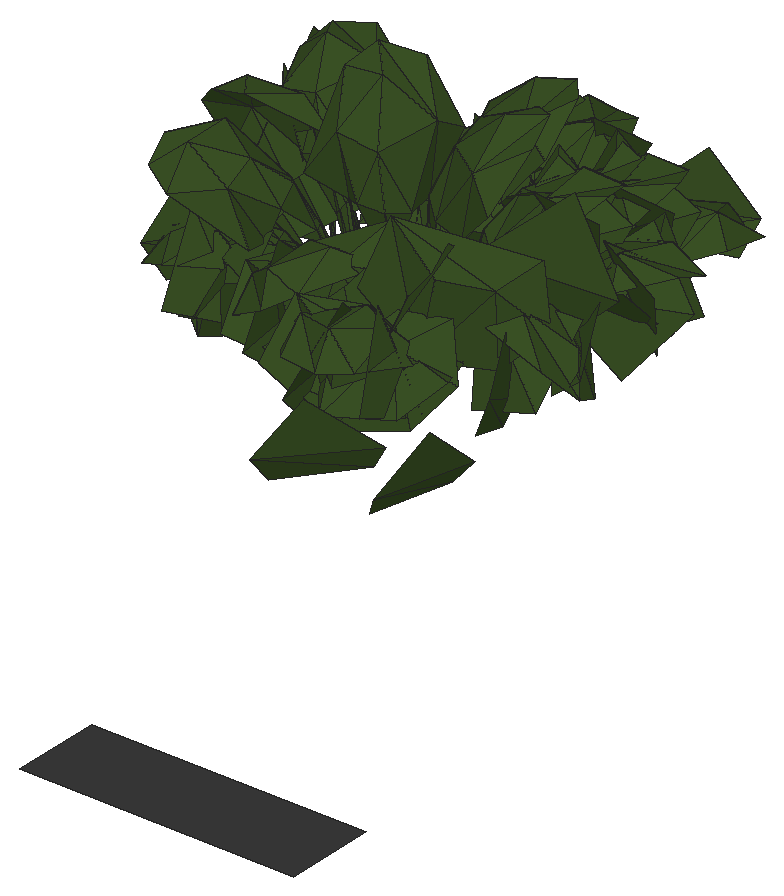
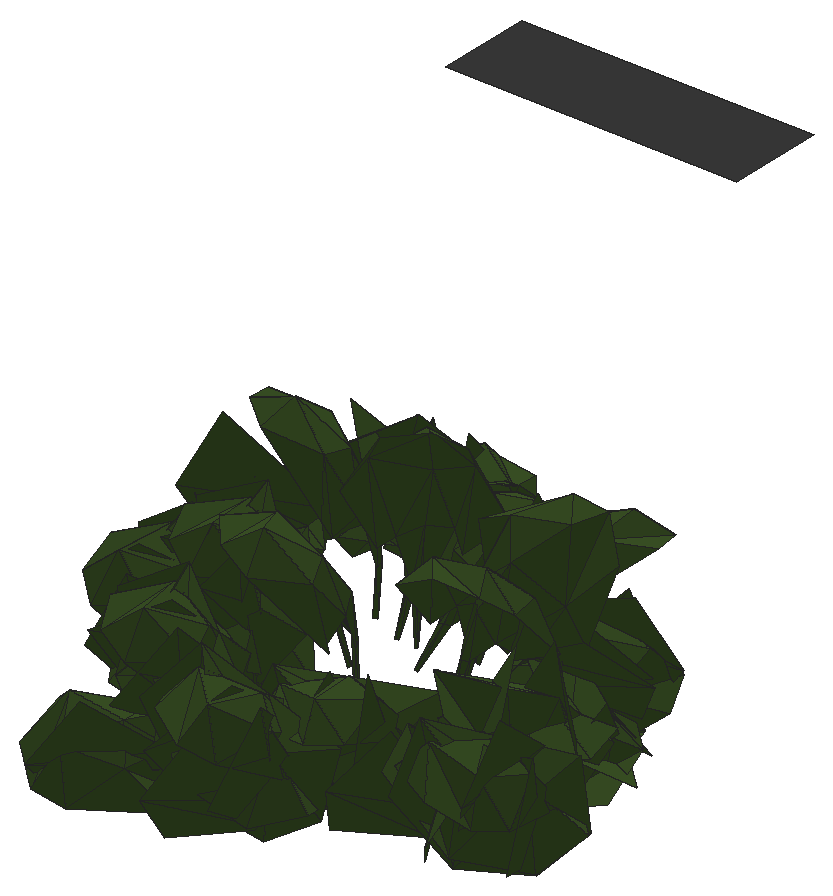
# SketchUp Ruby script. Lengths in inches.
U = 1.inch
M = Sketchup.active_model
def pt(a) = Geom::Point3d.new(a.map { |v| v * U })
def face(e, loops, mat)
  f = e.add_face(loops[0].map { |a| pt(a) })
  loops[1..].each { |l| e.add_face(l.map { |a| pt(a) }).erase! }
  f.material = f.back_material = mat if mat
  f
end
# faces: each face lists its corners as indices into pts; further lists are holes
def faces(e, pts, list, mat = nil) = list.each { |f| face(e, (f[0].is_a?(Array) ? f : [f]).map { |l| l.map { |i| pts[i] } }, mat) }
# xy, xz, yz: faces in a plane at the given z, y or x. An outline is a flat list of corners, or four numbers for a rectangle; further outlines are holes
def ring(l) = l.size == 4 ? [[l[0], l[1]], [l[2], l[1]], [l[2], l[3]], [l[0], l[3]]] : l.each_slice(2).to_a
def flat(e, list, mat, &to3) = list.each { |f| face(e, (f[0].is_a?(Array) ? f : [f]).map { |l| ring(l).map { |u, v| to3.(u, v) } }, mat) }
def xy(e, z, list, mat = nil) = flat(e, list, mat) { |x, y| [x, y, z] }
def xz(e, y, list, mat = nil) = flat(e, list, mat) { |x, z| [x, y, z] }
def yz(e, x, list, mat = nil) = flat(e, list, mat) { |y, z| [x, y, z] }
def lines(e, pts, list) = list.each { |a, b| e.add_line(pt(pts[a]), pt(pts[b])) }
# prism: a flat outline (further loops are holes) pulled along v
def prism(e, loops, v, mat = nil)
  f = face(e, loops, mat); d = Geom::Vector3d.new(v.map { |x| x * U })
  f.pushpull(f.normal.samedirection?(d) ? d.length : -d.length)
end
def box(e, o, s, mat = nil) = prism(e, [[o, [o[0] + s[0], o[1], o[2]], [o[0] + s[0], o[1] + s[1], o[2]], [o[0], o[1] + s[1], o[2]]]], [0, 0, s[2]], mat)
def at(x, y, z, deg = 0) = Geom::Transformation.translation(pt([x, y, z])) * Geom::Transformation.rotation(ORIGIN, Z_AXIS, deg.degrees)
def axes(o, x, y, z) = Geom::Transformation.new([*x, 0, *y, 0, *z, 0, *pt(o).to_a, 1])
def part(name) = M.definitions.add(name)
# library, detail: a bought-in or finely detailed component or shape, given as its bounding box
def library(name, o, s) = part(name).tap { |d| box(d.entities, o, s) }
def detail(e, o, s) = box(e.add_group.entities, o, s)
def put(e, d, t, mat = nil) = e.add_instance(d, t).tap { |i| i.material = mat if mat }
def group(e, t, mat = nil) = e.add_group.tap { |g| g.transformation = t; g.material = mat if mat }.entities
root = M.entities
M.materials.add("AM113_062_Tilia").color = [58, 81, 37]
M.materials.add("[Color M07]").color = [58, 58, 58]
xy(root,690.29,[[622.42,139.5,935.92,242.3125]],"[Color M07]")
p = [[327.63,1139.99,685.84],[309.71,1220.66,616.22],[297.98,1281.88,690],[174.23,954.27,619.67],[231,919.16,655.06],[205.29,943.34,722.98],
  [154.57,967.09,702.43],[140.39,1031,708.31],[108.83,998.61,649.08],[307.93,1122,668.52],[310.69,1104.29,621.81],[311.32,1108.2,619.89],
  [311.49,1128.11,668.52],[303.43,1122.55,663.09],[308.5,1107.52,620.19],[389.02,759.99,653.48],[390.55,785.18,622.06],[464.66,843.46,635.39],
  [420.88,1218.61,654.95],[420.67,1190.75,623.84],[419.95,1187.76,627.35],[395.14,1156.22,667.875],[395.59,1141.64,624.24],[393.67,1138.13,625.47],
  [83.33,1185.82,624.62],[56.51,1146.41,657.09],[82.44,1189.61,706.24],[130.1,1239.65,638.93],[395.65,1152.44,674.15],[397.61,1139.62,624.95],
  [402.38,1152.74,676.91],[423.08,1217.59,662.28],[423.24,1189.62,624.87],[429.7,1220.08,662.4375],[381.2,1345.93,663.1875],[365.77,1332.66,626.33],
  [280.68,1294.44,648.45],[550.8,901.41,709.43],[536.91,899.74,667.9375],[501.37,982.28,628.85],[500.73,1003.03,649.21],[185.51,1160.68,715.51],
  [167.09,1230.71,629.01],[121.44,1288.29,683.09],[187.5,1196.21,629.25],[174.67,1183.04,653.09],[228.74,1287.03,699.15],[233.375,1276.51,656.4],
  [70.38,1206.76,751.58],[90.97,1167.86,632.32],[164.75,1148.38,699.71],[70.45,1240.96,653.14],[413.95,1326.36,673.74],[381.95,1306.6875,632.77],
  [411.5625,1271.92,633.99],[447.59,1363.01,639.1875],[382.33,938.86,709.29],[393.79,860.28,633.7],[399.17,794.95,702.68],[562.03,1126.64,659.14],
  [518.35,1180.6,633.72],[509.52,1180.36,714.6875],[478.72,1212.45,656.82],[533.04,757.23,664.18],[513.99,775.86,634.76],[535.22,868.29,634.04],
  [552.33,878.07,656.07],[408.8,1270.31,671.65],[155.32,950.27,634.76],[208.75,906.27,669.96],[209.82,955.9375,720.57],[179.46,1062.71,668.15],
  [120.11,1023.59,651.5],[169,992.7,700.77],[147.91,1120.65,634.8],[83.88,1089.46,650.38],[108.71,1011.38,661.23],[136.75,1065.66,699.34],
  [176.39,1030.09,725.68],[247.48,1021.8125,698.34],[480.53,841.21,661.92],[325.08,1197.39,676.07],[332.71,1179.9,635.42],[333.03,1176.14,637.49],
  [298.78,993.79,708.55],[327.84,918.16,635.86],[309.45,849.57,695.18],[275.48,1041.15,635.88],[245.66,1034.51,674.23],[252.27,1034.3,677.43],
  [278.5,1042.57,639.24],[327.67,1195.35,682.82],[335.52,1179.4,636.17],[333.19,1199.55,684.54],[520.78,1189.57,764.04],[498.7,1175.5,636.34],
  [459.35,1104.71,693.92],[569.19,1185.41,676.24],[255.2,1029.8,673.47],[277.17,1039.02,637.22],[285.36,1300.09,637.23],[239.24,1281.06,663.58],
  [285.0625,1291.0625,718.17],[354.96,1310.96,657.4375],[448.375,1097.28,678.25],[437.37,1080.01,638.73],[434.24,1077.97,640.92],[113.56,1236.78,724.35],
  [169.17,1235.62,769.29],[162.83,1285.08,716.625],[467.15,1346.8,686.42],[482.3125,1367.17,647.91],[488.72,1366.5625,669],[485.34,1340.26,639.38],
  [407.73,1287.54,657.32],[447.81,1094.35,685.24],[438.32,1077.37,639.72],[454.17,1091.73,687.29],[285.01,1304.65,767.97],[280.18,1280.45,639.78],
  [324.8125,1210.37,692.13],[308.38,1345.99,679.18],[67.85,1205.9,640.49],[47.12,1160.9,665.06],[94.26,1183.34,708.76],[122.28,1254.76,658.12],
  [348.37,1204.82,707.76],[378.88,1283.14,641.04],[376.96,1346.91,712.72],[124.99,1008.1875,641.44],[182.85,975.625,677.9],[171.24,1019.73,734.7],
  [113.64,1107.77,694.77],[70.23,1067.42,662.12],[120.66,1044.59,715.81],[281.19,1237.625,642.22],[220.04,1199.44,646.54],[240.28,1194.91,723.81],
  [286.29,1230.3,729.59],[347.3,1210.41,747.36],[342.74,1264.82,703.2],[466.02,1082.3125,711.53],[549.87,1091.34,645.39],[603.58,1128.0625,715.14],
  [441.98,1023.9,736.48],[479.3125,965.46,645.89],[560.48,955.8125,674.03],[402.16,972.05,646.15],[399.66,950.03,693.13],[403.75,955.78,693.65],
  [403.11,975.8,648.38],[408.24,955.09,688.24],[405.03,972.46,646.53],[192.5,1165.17,686.79],[495.4,1297.59,708.6875],[514.02,1341.27,670.84],
  [271.59,1292.72,679.9],[411.16,1257.73,780.51],[404.89,1253.14,648.81],[400.51,1165.51,686.49],[460.25,1288.15,702.5],[521.99,960.06,741.96],
  [245.33,1209.74,772.58],[223.73,1179.5,649.5],[301.47,1135.125,679.47],[231.03,1252.6,681.81],[482.41,1235.93,674.75],[419.9375,1266.85,650.66],
  [408.1,1251.43,728.49],[368.9,1273.55,671.32],[174.04,1136.39,687.26],[193.76,1122.12,651.58],[196.14,1119.7,654.56],[149.86,1087.9,725.7],
  [104.32,1050.1,700.87],[162,1041.35,652.08],[238.74,1163.21,699.8125],[176.82,1137.3125,694.29],[196.22,1123.5625,652.34],[178.49,1144.17,694.7],
  [206.1,1228.36,738.91],[415.99,1146.52,701.32],[488.98,1201.49,653.22],[515.44,1248.21,737.56],[430.64,785.71,718.13],[397.04,1061.99,697.77],
  [397.28,1047.24,654.22],[394.88,1044.02,655.33],[228.125,1119.78,672.11],[150.4,1179.01,654.22],[119.5,1191.48,754.53],[425.14,1255.45,693],
  [260.47,913.6,712.85],[396.8,1058.21,704.08],[399,1044.97,655.06],[403.4,1057.64,707.27],[574.78,1132.12,682.14],[537.48,1192.99,655.09],
  [501.4375,1169.52,715.01],[492.82,1219.65,668.76],[150.6875,1034.22,776.35],[199.36,987.61,676.91],[207.05,1078.21,655.21],[571.36,1026.58,662.9],
  [508.7,1086.11,655.16],[536.35,1061.95,697.4],[477.6875,1054.83,670.76],[557.33,807.1,719.35],[450.28,1190.83,710.05],[142.6,1086.8125,785.74],
  [86.45,1129.4,727.68],[119.39,1085.28,657.11],[210.48,1100.67,662.48],[80.24,1129.95,716.82],[141.93,1013.26,700.02],[136.46,1025.74,657.22],
  [113.02,969.36,675.82],[195.45,1029.98,659.3],[392.23,1291.91,683.78],[338.14,1305.72,742.58],[380.23,1264.2,779.34],[406.84,1314.1875,739.65],
  [136.15,1218.42,729.85],[209.35,1201.64,734.37],[183.6,1268.87,726.67],[355.76,867.78,764.9375],[355.96,815.32,716.65],[420.39,839.65,658.67],
  [414.95,843.35,746.38],[464,874.67,743.95],[484.63,871.92,666.72],[532.64,1087.58,783.98],[589.65,1087.3,745.22],[548.27,1142.8,742.9],
  [285.11,1322.52,659.25],[240.54,1296.69,675.83],[290.47,1278.67,717.74],[357.62,1324.4,680.62],[210.99,1032.11,691.21],[440.25,1174.625,660.27],
  [499.62,1052.83,739.24],[162.5,971.05,702.34],[406.06,1238.26,725.55],[352.6,1222.62,661.45],[457.98,1132.11,729.83],[377.32,1284.57,686.8],
  [449.84,1244.37,687.74],[580.01,994.07,678],[563.32,1013.02,716.66],[298.69,1145.56,716.17],[271.88,1149.26,709.2],[345.79,1314.4375,729.71],
  [337.22,1028.22,663.36],[320.07,1004.35,703.1875],[323.97,1009.73,706.26],[337.62,1031.77,666.28],[246.45,1244.85,715.42],[177.58,943.39,761.84],
  [172.4,905.39,665.98],[245.28,932.07,663.82],[241.11,1022.99,684.89],[365.47,1171.22,695.2],[359.39,1242.97,702.7],[283.1,1252.11,664.45],
  [302.875,1206.4,723.91],[215.625,1220.98,669.27],[249.8125,1185.63,720.68],[253.15,1228.87,664.59],[391.88,1219,732.43],[329.68,1008.95,703.36],
  [339.78,1028.4,665.15],[99.08,1114.91,670.82],[103.73,1096.625,665.53],[113.05,1044.93,681.16],[137.76,1086.71,733.32],[124.36,1163.95,685.89],
  [514.66,901.65,709.91],[474.21,1246.19,666.9],[520.73,1279.89,685.1875],[398.93,1175.375,723.57],[390.23,1199.51,710.45],[283.85,962.29,711.39],
  [321.1875,1154.58,699.76],[446.01,1346.3125,735.66],[120.38,940.58,701.58],[143.73,948.17,669.27],[229.05,972.22,712.77],[190.07,1180.63,699.14],
  [254.5,922.49,739.52],[266.38,872.46,689.4],[344.11,894.48,669.56],[313.5,894.5625,748.34],[361.04,922.17,773.12],[402.66,921.4,711.46],
  [245.27,904.79,719.63],[480.54,1062.8,707.03],[457.08,858.12,791.4],[468.55,818.42,697.62],[482.7,891.94,671.1875],[408.89,941.65,703.625],
  [343.42,1103.42,717.35],[349.5,1096.53,671.32],[348.35,1092.59,671.41],[351.27,1234.43,714.82],[344.42,1098.9,722.64],[351.88,1094.89,671.83],
  [436.0625,1299.49,701.18],[350.75,1100.125,726.39],[160.7,1117.14,787.75],[223.67,1017.62,716.31],[233.88,991.98,716.29],[554,1030.27,735.92],
  [458.4,1232.23,757.11],[468.44,1171.22,785.5],[520.77,1202.13,757.84],[479.27,1144.55,675.53],[468.32,1141.6,710.47],[506.66,1178.97,732.97],
  [479.56,1189.95,681.94],[130.07,929.46,689.27],[261.125,1158.63,676.08],[246.03,1192.86,740.81],[83.68,1189.81,724.9],[77.95,1154.2,681.75],
  [123.13,1159.32,676.08],[126.53,1154.42,713.18],[220.15,1164.65,700.96],[318.71,1222.5,727.26],[298.0625,1236.16,711.51],[582.7,990.76,699.98],
  [552.82,988.02,676.53],[495.56,1063,688.98],[332.55,1219.35,737.28],[331.53,1175.36,676.71],[353.32,1227.08,700.89],[299.26,1247.66,676.68],
  [285.72,1287.61,736.35],[260.35,1270.28,686.79],[126.4,975,706.9375],[421.34,1160.52,716.91],[429.87,1283.36,677.1875],[489.88,1243.3,700.5625],
  [220.55,980.67,727.2],[520.62,985.08,755.66],[560.62,964.46,713.07],[466.51,1117.73,728.18],[400.29,1211.88,678.63],[405.29,1246.38,745.6875],
  [378.9,1250.79,692.4375],[248.27,1061.41,723.88],[259.68,1064.92,678.92],[262.64,1062.08,679.14],[252.44,1060.0625,729.51],[262.19,1066.26,679.72],
  [421.81,1161.11,811.29],[420.2,1156.68,679.35],[402.84,1070.59,716.71],[225.44,1122.75,679.42],[477.5,1184.4,736.64],[341.75,910.78,715.72],
  [341.33,838.56,717.66],[416.94,824.39,679.7],[400.63,868.86,742.39],[455.36,884.9,741.43],[486.86,849.05,687.77],[254.05,1066.13,733.7],
  [344.56,1277.03,741],[413.03,1287.5625,743.23],[264.52,1068.73,680.92],[243.01,1076.87,727.22],[249.6875,1079.17,727.33],[267.35,1071.86,681.41],
  [162.95,1035.87,707.13],[428.9,1044.99,705.28],[397.63,1038.8125,681.42],[395.07,1039.8125,685.35],[253.31,1074.23,726.22],[266.91,1067.93,682.8125],
  [69.16,1239.67,696.18],[561.46,1186.56,718.14],[569.55,1068.9375,749.96],[526.53,1122.97,742.56],[493.66,1129.57,710.4],[436.83,1168.3,682.2],
  [420.01,1154.99,759.15],[386.37,1181.76,699.45],[100.04,1225.16,758.79],[429.03,1043.8,713.1],[396.9,1036.37,683.24],[432.16,1037.51,714.13],
  [349.01,1013.16,732.16],[339.85,1026.48,684.39],[338.9,1030.13,686.86],[343.15,1014.08,729.91],[336.67,1028.25,686.84],[345.48,1221.29,720.04],
  [199.96,950.29,737.93],[245.3,938.87,718.22],[239.59,976.25,685.16],[258.05,968.6,691.9],[253.66,896.65,685.76],[334.02,878.59,685.68],
  [302.65,921.23,740.47],[354.28,933.11,767.73],[397.44,897.51,729.52],[279.17,1219.08,767.29],[151.07,1139.32,760.52],[212.13,1162.69,767.99],
  [165.85,1206.97,758.76],[223.92,1137.23,731.66],[305.56,1339.2,721.22],[350.79,1018.59,737.53],[478.78,1093.57,723.14],[149.9,1158.71,731.28],
  [515.56,885.5,721.06],[410.3,929.33,739.48],[436.75,923.5625,732.55],[416.37,1142.18,756.08],[363.92,1133.37,688.52],[453.64,1030.16,763.82],
  [395.55,1191.66,715.47],[501.62,1082.28,710.24],[161.97,918.08,703.5],[143.875,956.35,721.44],[415.08,1049.81,732.55],[496.48,1094.45,689.34],
  [525.5,1137.74,775.3125],[294.24,960.63,690.51],[261.45,911.375,690.57],[270.1,912.22,735.46],[298.85,977.18,721.11],[288.92,860.66,722.42],
  [190.01,989.72,733.98],[92.13,1274.36,725.21],[108.94,1258.25,691.37],[110.43,1163.79,702.03],[395.84,994.41,755.82],[450.75,1279.85,742.41],
  [266.89,1010.03,735.16],[272.52,1025.38,692.57],[274.88,1028.47,694.25],[387.29,923.14,722.11],[270.82,1027.7,693.13],[259.63,1014.51,743.39],
  [266.5,1013.71,741.55],[172.29,1173.25,723.47],[229.41,1032.31,746.875],[309.67,900.96,788.62],[97.93,1244.7,739.59],[86.02,1270.35,704.6],
  [84.85,1025.19,734.64],[102.93,1020.18,696.41],[195.29,1040.14,706.86],[458.57,915.9,710.98],[510.39,964.86,696.55],[508.61,963.57,778.27],
  [539.73,1002.72,728.48],[445.75,1010.28,773.91],[518.37,1040.8,697.21],[587.1,1040.91,760.83],[375.4,904.47,697.36],[348.82,853.89,717.18],
  [369.77,858.03,754.35],[515.61,1042.32,734.96],[401.12,1080.78,753.64],[396.2,1105.77,739.95],[91.96,1101.68,697.91],[121.51,1168.79,714.125],
  [206.07,976.66,740.77],[381.5,1026.86,698.3],[381.45,1021.53,749.96],[382.16,1027.14,746.72],[385.65,1027.52,698.85],[384.08,1029.93,699.4],
  [408.39,1001.82,780.82],[422.84,927.78,698.73],[461.53,868.1,757.83],[447.02,914.82,698.9],[458.26,876.43,761.01],[486.99,904,723.76],
  [387.83,1019.43,752.78],[362.05,1145.53,741.73],[176.88,1136.375,742.67],[285.5,1183.2,745.24],[191.53,1204.04,746.73],[566.9,1040.74,759.89],
  [448.59,1205.11,749.54],[511.44,1176.33,755.8],[310.66,1269.58,723.6],[240.03,1247.27,722.74],[436.85,1234.1,787.7],[232.97,974.59,745.89],
  [149.55,970.04,774.4],[100.72,1152.18,729.42],[156.2,1239.67,752.28],[182.44,1195.39,702.47],[182.62,1251.87,725.22],[422.61,852.12,784.97],
  [315.32,980.82,748.92],[372.89,1277.8,765.22],[367.57,1235.39,703.17],[401.85,1275.29,738.11],[341.52,973.41,754.68],[470.73,1187.89,774.32],
  [448.8,1161.86,703.88],[495.9375,1172.76,747.82],[127.19,1281.15,721.92],[470.26,1048.8,734.69],[485.71,947.13,705.47],[204.78,1050.27,735.34],
  [421.61,1063.07,748.47],[502.14,1080.57,707.69],[553.4,1072.3,744.28],[540.97,1099.98,768.96],[319.53,1299.72,775.42],[258.3,956.94,755.53],
  [409.04,1116.54,708.84],[415.89,1150.45,776.13],[392.45,1158,721.21],[501.01,1136.03,736.67],[447.79,1183.51,709.34],[485.34,930.18,756.51],
  [466.15,1129.49,791.06],[466.94,1067.85,820.1],[523.91,1091.46,795.93],[416.07,1208.28,758.26],[500.29,1141.86,753.18],[416.35,927.47,838.93],
  [419.68,876.03,789.03],[472.86,919.96,796.99],[419.14,946.77,769.03],[533.5,1157.57,774.34],[315.71,1263.41,753.59],[502.83,955.67,742.45],
  [120.71,1191.92,746.78],[461.2,1023.06,737.53],[387.26,806.76,737.03],[339.8,1113.63,776.86],[326.7,1137.06,768.56],[555.71,1157.06,760.59],
  [587.64,1165.49,733.37],[314.46,939.14,773.43],[465.43,1177.64,775.86],[330.3125,1318.97,761.27],[337.5,1351.3,734.24],[419.75,889.375,765.7],
  [462.8,996.32,722.23],[329.02,851.3125,744.62],[278.12,1240.3,751.17],[266.08,1271.5,724.83],[459.6,822.64,738.78],[234.31,1061.22,782.29],
  [208.01,1060.64,771.54],[91.23,1224.67,788.86],[232.36,1079.85,780.58],[249.59,1061.1875,794.52],[365.25,1105.03,770.07],[213.09,1077.71,755.65],
  [360.47,965.46,727.61],[350.81,923.57,786.3],[389.61,950.55,768.71],[515.9,1023.08,786.11],[415.93,930.11,778.03],[351.53,999.98,787.26],
  [324.89,993.25,790.69],[443.85,1134.35,820.18],[589.85,1123.09,751.11],[253.95,1080.02,778.16],[376.19,1331.97,748.45],[127.9,1066.7,781.64],
  [255.33,990.65,788.92],[260.89,965.67,775.6],[313.3,881.46,769.74],[453.17,1103.87,782.86],[511.36,1067.11,793.28],[431.47,800.79,738.65],
  [471.84,1084.02,809.08],[449.49,1060.72,737.28],[495.85,1065.5625,784.28],[363.82,1024.08,781.86],[195.24,1058.9,738.07],[140.66,1045.81,762.22],
  [154.68,1056.68,802.4375],[421.95,831.67,767.24],[379.71,975.24,800.96],[421.05,1111.32,789.41],[235.32,921.36,805.96],[264.85,913.59,756.21],
  [251.58,955.88,741.96],[335.5,1156.02,741.95],[329.01,1179.35,816.41],[305.3,1186.72,761.63],[457.35,1245.6,778.18],[482.91,1271.18,758.68],
  [236.43,1009.28,780.24],[356.02,870.9375,760.66],[196.67,1077.93,744.625],[168.95,1080.83,816.92],[154.57,1064.74,759.9],[384.07,1023.13,807.58],
  [380.87,1050.45,810.46],[503.84,1232.68,769.54],[404.07,1008.05,793.33],[211.05,1061.09,826.96],[185.42,896.29,794.87],[486.4,931.39,831.52],
  [148.1875,1132.54,828.99],[533.5,1045.25,852.01],[365.97,1221.15,827.92],[404.05,1132.1,839.93],[392.375,1113.98,761.71],[433.38,1126.97,814.125],
  [137.53,1006.6,825.26],[210.375,1012.95,763.65],[158.71,1009.41,800.57],[178.67,989.62,829.31],[347.25,1143.06,821.12],[209.21,1080.15,825.29],
  [243.89,1124.93,849.43],[258.89,1108.4375,771.57],[263.27,1149.31,826.47],[230.13,960.48,819.26],[466.04,1143,812.03],[495.48,1164.9,794.25],
  [232.59,1033.38,853.75],[276.33,1022,828.7],[255.89,1035.2,778.84],[303.11,992.62,857.66],[273.43,982.77,808.68],[302.42,1010.32,780.21],
  [341.3125,1002.81,844.76],[371.97,1050.92,867.27],[360.68,1053.06,785.6],[432.35,1008.19,783.49],[476.33,992.3125,830.26],[451.84,1001.17,862.08],
  [510.7,1124.04,806.49],[376.41,1083.24,848.04],[395.71,1070.38,790.27],[400.39,1075.37,870.53],[380.16,1103.52,825.52],[403.29,1035.73,858.71],
  [154.02,910.03,807.37],[181.75,930.41,831.54],[139.09,951.32,817.67],[167.06,983.99,857.1],[175.96,1022.14,858.25],[279.88,1032.33,899.97],
  [426.57,1182.46,850.86],[378.02,1184,855.57],[185.12,1125.33,859.77],[450.86,1096.13,889.41],[208.96,1167.8,859.23],[398.27,1216.79,846.4375],
  [202.2,986.39,863.89],[165.82,1158.65,850.41],[492.3,1034.78,886.16],[324.24,1031.74,905.37],[337.18,1078.51,910.9],[448.24,1052.45,900.24],
  [479.37,1076.24,899.43],[298.08,1058.38,920.73]]
faces(root,p,[[0,1,2],[3,4,5],[5,6,3],[7,8,3],[3,6,7],[9,10,11],[11,12,9],[13,14,10],
  [10,9,13],[15,16,17],[18,19,20],[21,22,23],[24,25,26],[27,24,26],[28,23,29],[29,30,28],
  [31,20,32],[32,33,31],[23,28,21],[34,35,36],[20,31,18],[37,38,39],[39,40,37],[41,42,43],
  [44,45,46],[46,47,44],[48,49,50],[48,51,49],[52,53,54],[55,53,52],[56,57,58],[59,60,61],
  [60,62,61],[63,64,65],[65,66,63],[54,67,52],[68,69,70],[71,72,68],[68,73,71],[70,73,68],
  [74,75,76],[76,77,74],[78,79,74],[74,77,78],[17,80,15],[81,82,83],[84,85,86],[87,88,89],
  [89,90,87],[91,83,92],[92,93,91],[94,95,96],[94,97,95],[98,99,90],[100,101,102],[103,100,102],
  [83,91,81],[104,105,106],[26,107,27],[27,107,108],[108,109,27],[90,89,98],[110,55,52],[111,55,110],
  [112,113,114],[115,106,116],[116,117,115],[118,119,120],[118,121,119],[122,123,124],[125,122,124],[106,115,104],
  [126,127,128],[129,130,131],[132,133,129],[129,134,132],[131,134,129],[135,136,137],[137,138,135],[139,140,135],
  [135,138,139],[141,142,143],[144,145,146],[147,148,149],[149,150,147],[151,152,150],[136,153,137],[111,110,154],
  [154,155,111],[150,149,151],[36,156,34],[157,158,159],[157,160,158],[40,161,37],[162,163,164],[162,165,163],
  [166,167,168],[167,169,168],[170,171,172],[173,174,175],[173,175,176],[177,172,178],[178,179,177],[45,180,46],
  [181,182,183],[80,184,15],[185,186,187],[188,189,190],[172,177,170],[18,31,191],[191,67,18],[4,192,5],
  [193,187,194],[194,195,193],[196,197,198],[197,199,198],[200,201,202],[203,204,205],[205,204,206],[187,193,185],
  [66,207,63],[61,62,208],[209,210,211],[209,211,212],[26,25,213],[214,215,216],[217,215,214],[114,218,112],
  [103,219,220],[220,221,103],[102,219,103],[124,222,125],[223,224,125],[125,222,223],[225,226,227],[227,228,225],
  [229,228,227],[227,230,229],[231,232,59],[59,233,231],[61,233,59],[234,235,236],[237,234,236],[214,238,217],
  [198,239,240],[198,199,239],[76,241,78],[78,77,76],[242,243,244],[242,245,243],[191,31,33],[33,246,191],
  [247,203,248],[248,203,205],[13,9,249],[249,250,13],[156,251,34],[252,253,254],[254,255,252],[102,101,256],
  [257,258,259],[257,259,260],[261,262,263],[263,264,261],[263,265,266],[266,264,263],[236,267,268],[236,235,267],
  [269,270,255],[124,123,271],[272,273,274],[275,272,274],[255,254,269],[230,276,229],[154,246,277],[277,278,154],
  [21,28,279],[279,280,21],[71,73,70],[70,281,71],[249,9,12],[12,282,249],[218,283,112],[284,285,286],
  [265,287,266],[288,289,290],[290,291,288],[292,291,290],[290,293,292],[69,294,70],[206,295,205],[124,271,223],
  [154,278,155],[296,297,298],[296,298,299],[300,301,302],[168,169,303],[302,304,300],[304,302,305],[306,67,191],
  [306,52,67],[305,307,304],[308,188,190],[309,310,98],[98,89,309],[306,110,52],[311,144,146],[88,238,309],
  [309,89,88],[279,28,30],[166,312,313],[313,314,166],[168,312,166],[315,316,317],[317,318,315],[214,216,319],
  [320,250,321],[322,323,324],[324,325,322],[321,326,320],[81,91,327],[327,328,81],[329,330,331],[332,282,333],
  [333,334,332],[335,328,336],[336,337,335],[200,338,201],[30,339,279],[340,245,242],[341,340,242],[130,342,131],
  [343,344,247],[247,248,343],[104,115,345],[345,316,104],[346,280,347],[347,348,346],[349,350,351],[351,352,349],
  [352,351,353],[354,355,356],[266,287,357],[266,357,261],[354,358,355],[359,360,361],[361,362,359],[363,362,361],
  [361,364,363],[353,365,352],[237,366,268],[268,367,237],[236,366,237],[368,369,370],[370,371,368],[274,273,372],
  [373,374,375],[376,377,371],[371,370,376],[378,323,322],[379,318,317],[240,380,196],[196,381,240],[198,381,196],
  [382,383,384],[383,385,384],[327,91,93],[386,41,43],[387,375,388],[388,389,387],[390,391,392],[391,390,393],
  [393,394,391],[93,395,327],[396,397,398],[398,310,396],[345,115,117],[375,387,373],[399,400,401],[401,402,399],
  [403,402,401],[401,404,403],[405,0,2],[274,406,275],[275,406,407],[407,408,275],[154,110,306],[137,153,409],
  [410,337,336],[392,411,390],[117,412,345],[413,325,170],[170,177,413],[306,191,246],[246,154,306],[364,414,363],
  [415,416,151],[151,149,415],[417,418,419],[417,420,418],[331,421,329],[319,422,423],[319,423,214],[424,425,426],
  [427,428,429],[429,430,427],[429,428,431],[238,214,432],[432,309,238],[433,434,435],[399,402,403],[403,436,399],
  [437,348,347],[438,439,440],[148,441,415],[415,149,148],[442,443,444],[444,440,442],[440,444,438],[413,177,179],
  [179,445,413],[131,446,132],[132,134,131],[447,84,86],[261,264,266],[448,378,322],[449,378,448],[450,451,452],
  [453,454,455],[454,456,455],[457,458,459],[460,461,462],[462,441,460],[463,248,205],[463,205,295],[185,193,464],
  [464,465,185],[466,174,173],[467,466,173],[78,468,79],[469,470,471],[470,469,472],[471,473,469],[474,475,476],
  [477,416,478],[478,479,477],[472,480,470],[384,385,481],[176,482,173],[467,482,176],[483,249,282],[282,332,483],
  [176,484,467],[214,423,432],[421,485,329],[341,486,244],[244,487,341],[242,486,341],[332,334,488],[489,326,321],
  [490,181,183],[286,491,284],[491,492,284],[435,493,433],[241,468,78],[7,6,5],[494,445,495],[495,496,494],
  [497,56,58],[253,430,498],[498,254,253],[499,395,500],[500,501,499],[498,502,269],[269,254,498],[423,422,396],
  [422,397,396],[503,339,504],[504,505,503],[464,193,195],[494,506,449],[449,448,494],[373,387,507],[507,295,373],
  [363,508,359],[363,414,508],[26,213,108],[108,107,26],[452,509,450],[463,295,507],[274,372,407],[195,510,464],
  [511,512,513],[513,412,511],[514,126,128],[5,515,7],[516,465,517],[517,518,516],[223,222,124],[483,250,249],
  [483,321,250],[519,520,417],[520,420,417],[229,276,521],[61,208,231],[382,522,523],[523,524,382],[384,522,382],
  [525,280,279],[525,347,280],[526,316,345],[526,317,316],[527,528,453],[453,529,527],[455,529,453],[70,294,281],
  [293,530,292],[531,141,143],[532,328,327],[532,336,328],[5,192,515],[343,533,344],[507,387,389],[534,322,325],
  [534,325,413],[389,535,507],[173,482,467],[231,233,61],[168,303,313],[240,381,198],[102,256,220],[359,362,363],
  [432,396,310],[432,310,309],[343,248,463],[525,279,339],[339,503,525],[462,461,536],[300,304,537],[537,538,300],
  [268,366,236],[539,379,317],[540,379,539],[220,219,102],[395,499,532],[532,327,395],[430,429,541],[541,498,430],
  [542,518,517],[543,410,336],[544,410,543],[432,423,396],[494,496,506],[441,462,545],[545,415,441],[546,533,343],
  [343,535,546],[429,431,547],[537,304,307],[548,489,321],[549,489,548],[526,345,412],[412,513,526],[534,413,445],
  [445,494,534],[332,488,549],[550,479,478],[137,409,139],[139,138,137],[349,352,551],[551,552,349],[549,548,332],
  [534,448,322],[493,553,433],[244,486,242],[554,555,376],[376,370,554],[307,556,537],[131,342,446],[369,557,554],
  [554,370,369],[558,502,559],[559,560,558],[455,456,561],[313,312,168],[404,562,403],[551,352,365],[563,564,393],
  [393,390,563],[563,390,411],[545,478,416],[545,416,415],[565,424,426],[526,539,317],[407,406,274],[513,566,540],
  [540,539,513],[365,567,551],[544,543,499],[499,568,544],[509,569,450],[463,507,535],[535,343,463],[570,571,438],
  [438,444,570],[547,572,429],[429,572,541],[532,543,336],[519,573,419],[419,574,519],[417,573,519],[462,536,575],
  [576,510,577],[577,578,576],[332,548,483],[411,579,563],[580,581,582],[582,557,580],[499,501,568],[575,583,462],
  [575,550,583],[583,550,478],[288,291,292],[292,584,288],[494,448,534],[585,465,464],[585,517,465],[483,548,321],
  [570,444,443],[384,481,523],[586,587,588],[588,571,586],[589,538,590],[590,591,589],[592,437,347],[593,437,592],
  [443,594,570],[225,228,229],[229,521,225],[513,512,566],[547,595,572],[596,552,597],[597,598,596],[525,592,347],
  [471,470,599],[599,600,471],[503,505,601],[585,464,510],[510,576,585],[541,502,498],[599,470,480],[480,602,599],
  [513,539,526],[499,543,532],[462,583,545],[541,559,502],[557,582,603],[603,554,557],[403,562,436],[419,573,417],
  [604,587,586],[605,474,476],[503,592,525],[593,592,503],[503,601,593],[523,522,384],[606,598,597],[572,595,559],
  [595,560,559],[607,457,459],[545,583,478],[608,591,590],[609,556,610],[610,611,609],[582,581,612],[613,614,615],
  [615,594,613],[616,538,537],[616,590,538],[292,530,584],[541,572,559],[616,537,556],[556,609,616],[617,597,552],
  [617,552,551],[618,567,619],[619,620,618],[621,586,571],[621,571,570],[622,542,517],[623,542,622],[585,622,517],
  [617,551,567],[567,618,617],[527,529,455],[455,561,527],[624,625,626],[626,555,624],[594,615,621],[621,570,594],
  [627,628,629],[629,564,627],[603,555,554],[630,563,579],[579,631,630],[631,579,632],[633,634,635],[635,602,633],
  [576,578,636],[632,637,631],[630,564,563],[576,622,585],[638,600,639],[639,640,638],[630,627,564],[602,635,641],
  [641,599,602],[623,622,576],[576,636,623],[603,624,555],[642,604,643],[643,604,586],[615,614,644],[582,612,645],
  [645,646,582],[582,646,603],[621,643,586],[615,644,642],[642,643,615],[641,600,599],[647,628,627],[641,639,600],
  [609,611,648],[616,649,590],[649,608,590],[617,650,597],[650,606,597],[615,643,621],[609,649,616],[618,650,617],
  [651,640,639],[618,620,652],[603,646,624],[653,608,649],[654,625,624],[655,606,650],[635,634,656],[653,649,609],
  [609,648,653],[630,657,627],[631,657,630],[631,637,658],[618,652,655],[655,650,618],[646,654,624],[645,654,646],
  [657,647,627],[635,659,641],[641,659,639],[660,659,635],[635,656,660],[661,657,631],[631,658,661],[659,651,639],
  [660,651,659],[661,647,657]],"AM113_062_Tilia")
